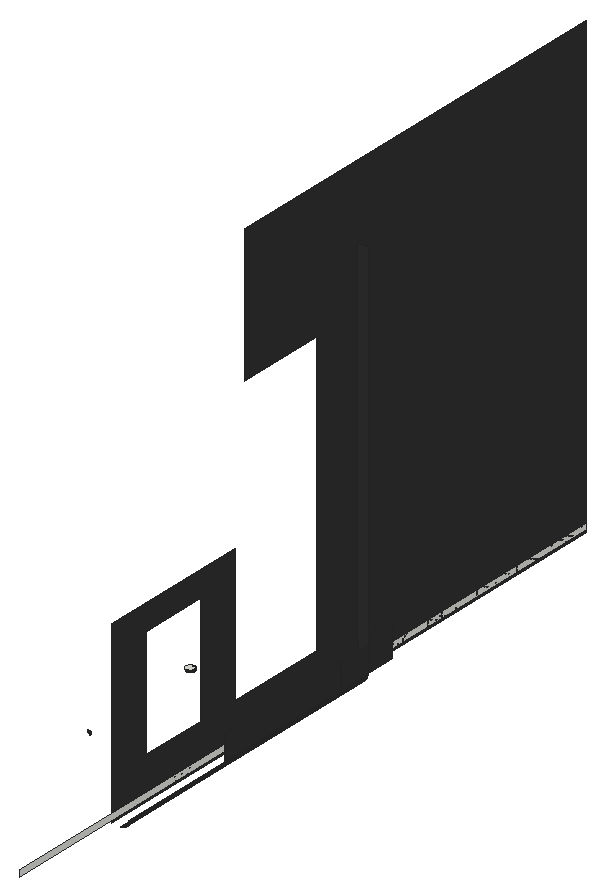
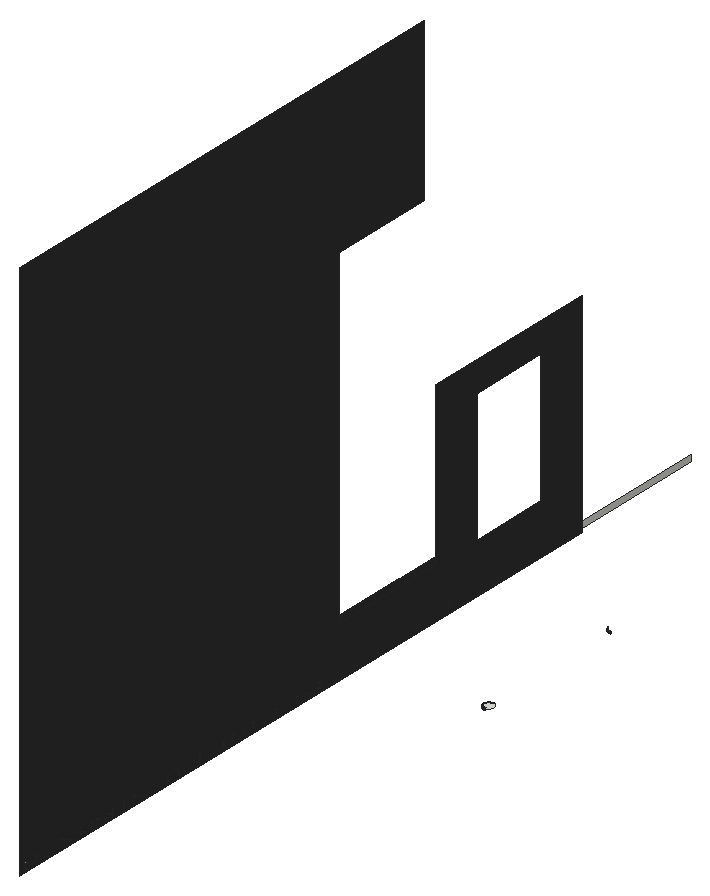
# SketchUp Ruby script. Lengths in inches.
U = 1.inch
M = Sketchup.active_model
def pt(a) = Geom::Point3d.new(a.map { |v| v * U })
def face(e, loops, mat)
  f = e.add_face(loops[0].map { |a| pt(a) })
  loops[1..].each { |l| e.add_face(l.map { |a| pt(a) }).erase! }
  f.material = f.back_material = mat if mat
  f
end
# faces: each face lists its corners as indices into pts; further lists are holes
def faces(e, pts, list, mat = nil) = list.each { |f| face(e, (f[0].is_a?(Array) ? f : [f]).map { |l| l.map { |i| pts[i] } }, mat) }
# xy, xz, yz: faces in a plane at the given z, y or x. An outline is a flat list of corners, or four numbers for a rectangle; further outlines are holes
def ring(l) = l.size == 4 ? [[l[0], l[1]], [l[2], l[1]], [l[2], l[3]], [l[0], l[3]]] : l.each_slice(2).to_a
def flat(e, list, mat, &to3) = list.each { |f| face(e, (f[0].is_a?(Array) ? f : [f]).map { |l| ring(l).map { |u, v| to3.(u, v) } }, mat) }
def xy(e, z, list, mat = nil) = flat(e, list, mat) { |x, y| [x, y, z] }
def xz(e, y, list, mat = nil) = flat(e, list, mat) { |x, z| [x, y, z] }
def yz(e, x, list, mat = nil) = flat(e, list, mat) { |y, z| [x, y, z] }
def lines(e, pts, list) = list.each { |a, b| e.add_line(pt(pts[a]), pt(pts[b])) }
# prism: a flat outline (further loops are holes) pulled along v
def prism(e, loops, v, mat = nil)
  f = face(e, loops, mat); d = Geom::Vector3d.new(v.map { |x| x * U })
  f.pushpull(f.normal.samedirection?(d) ? d.length : -d.length)
end
def box(e, o, s, mat = nil) = prism(e, [[o, [o[0] + s[0], o[1], o[2]], [o[0] + s[0], o[1] + s[1], o[2]], [o[0], o[1] + s[1], o[2]]]], [0, 0, s[2]], mat)
def at(x, y, z, deg = 0) = Geom::Transformation.translation(pt([x, y, z])) * Geom::Transformation.rotation(ORIGIN, Z_AXIS, deg.degrees)
def axes(o, x, y, z) = Geom::Transformation.new([*x, 0, *y, 0, *z, 0, *pt(o).to_a, 1])
def part(name) = M.definitions.add(name)
# library, detail: a bought-in or finely detailed component or shape, given as its bounding box
def library(name, o, s) = part(name).tap { |d| box(d.entities, o, s) }
def detail(e, o, s) = box(e.add_group.entities, o, s)
def put(e, d, t, mat = nil) = e.add_instance(d, t).tap { |i| i.material = mat if mat }
def group(e, t, mat = nil) = e.add_group.tap { |g| g.transformation = t; g.material = mat if mat }.entities
root = M.entities
M.materials.add("[Granite Dark Gray]").color = [51, 50, 50]
xy(root,126,[[438,183,438.11,393],[438.11,183,438.22,393]],"[Granite Dark Gray]")
xy(root,129,[[359.84,339,359.76,339.01,359.6875,339.02,359.61,339.03,359.45,339.05,359.375,339.07,359.3,339.08,359.22,339.1,359.15,339.125,359.07,339.15,359,339.17,358.92,339.2,358.71,339.29,358.64,339.33,358.57,339.36,358.43,339.44,358.37,339.48,358.3,339.53,358.24,339.57,358.17,339.62,357.93,339.82,357.88,339.88,357.82,339.93,357.62,340.17,357.57,340.24,357.53,340.3,357.48,340.37,357.44,340.43,357.36,340.57,357.33,340.64,357.29,340.71,357.2,340.92,357.17,341,357.15,341.07,357.125,341.15,357.1,341.22,357.08,341.3,357.07,341.375,357.05,341.45,357.03,341.61,357.02,341.6875,357.01,341.76,357,341.84,357,342.16,357.01,342.24,357.02,342.3125,357.03,342.39,357.05,342.55,357.07,342.625,357.08,342.7,357.1,342.78,357.125,342.85,357.15,342.93,357.17,343,357.2,343.08,357.29,343.29,357.33,343.36,357.36,343.43,357.44,343.57,357.48,343.63,357.53,343.7,357.57,343.76,357.62,343.83,357.82,344.07,357.88,344.12,357.93,344.18,358.17,344.38,358.24,344.43,358.3,344.47,358.37,344.52,358.43,344.56,358.57,344.64,358.64,344.67,358.71,344.71,358.92,344.8,359,344.83,359.07,344.85,359.15,344.875,359.22,344.9,359.3,344.92,359.375,344.93,359.45,344.95,359.61,344.97,359.6875,344.98,359.76,344.99,359.84,345,360.16,345,360.24,344.99,360.3125,344.98,360.39,344.97,360.55,344.95,360.625,344.93,360.7,344.92,360.78,344.9,360.85,344.875,360.93,344.85,361,344.83,361.08,344.8,361.29,344.71,361.36,344.67,361.43,344.64,361.57,344.56,361.63,344.52,361.7,344.47,361.76,344.43,361.83,344.38,362.07,344.18,362.12,344.12,362.18,344.07,362.38,343.83,362.43,343.76,362.47,343.7,362.52,343.63,362.56,343.57,362.64,343.43,362.67,343.36,362.71,343.29,362.8,343.08,362.83,343,362.85,342.93,362.875,342.85,362.9,342.78,362.92,342.7,362.93,342.625,362.95,342.55,362.97,342.39,362.98,342.3125,362.99,342.24,363,342.16,363,341.84,362.99,341.76,362.98,341.6875,362.97,341.61,362.95,341.45,362.93,341.375,362.92,341.3,362.9,341.22,362.875,341.15,362.85,341.07,362.83,341,362.8,340.92,362.71,340.71,362.67,340.64,362.64,340.57,362.56,340.43,362.52,340.37,362.47,340.3,362.43,340.24,362.38,340.17,362.18,339.93,362.12,339.88,362.07,339.82,361.83,339.62,361.76,339.57,361.7,339.53,361.63,339.48,361.57,339.44,361.43,339.36,361.36,339.33,361.29,339.29,361.08,339.2,361,339.17,360.93,339.15,360.85,339.125,360.78,339.1,360.7,339.08,360.625,339.07,360.55,339.05,360.39,339.03,360.3125,339.02,360.24,339.01,360.16,339]])
xy(root,132,[[443.875,267,444,268],[443.875,303,444,304],[443.875,369,444,370]],"[Granite Dark Gray]")
xz(root,252,[[359.84,128,359.92,129],[359.92,128,360,129],[360,128,360.08,129],[360.08,128,360.16,129]])
xz(root,267,[[443.875,132,444,150]],"[Granite Dark Gray]")
xz(root,268,[[443.875,132,444,150]],"[Granite Dark Gray]")
xz(root,303,[[443.875,132,444,150]],"[Granite Dark Gray]")
xz(root,304,[[443.875,132,444,150]],"[Granite Dark Gray]")
xz(root,339,[[359.84,128,359.92,129],[359.92,128,360,129],[360,128,360.08,129],[360.08,128,360.16,129]])
xz(root,345,[[359.84,128,359.92,129],[359.92,128,360,129],[360,128,360.08,129],[360.08,128,360.16,129]])
xz(root,369,[[443.875,132,444,150]],"[Granite Dark Gray]")
xz(root,370,[[443.875,132,444,150]],"[Granite Dark Gray]")
xz(root,393,[[437,126,437,150,436.875,150,436.875,151,437,151,437,210,436.875,210,436.875,211,437,211,437,234,436.875,234,436.875,235,437,235,437,294,436.875,294,436.875,295,437,295,437,378,436.875,378,436.875,379,437,379,437,402,444,402,444,363,443.875,363,443.875,362,444,362,444,333,443.875,333,443.875,332,444,332,444,279,443.875,279,443.875,278,444,278,444,249,443.875,249,443.875,248,444,248,444,200,443.875,200,443.875,199,444,199,444,151,443.875,151,443.875,150,444,150,444,131.78,443.95,131.23,443.93,131.12,443.92,131.01,443.9,130.9,443.85,130.68,443.83,130.57,443.8,130.46,443.77,130.36,443.74,130.25,443.71,130.15,443.67,130.04,443.63,129.9375,443.59,129.83,443.47,129.53,443.27,129.13,443.21,129.03,443.16,128.9375,443.1,128.84,442.98,128.66,442.92,128.5625,442.85,128.47,442.79,128.38,442.72,128.3,442.65,128.21,442.51,128.04,442.43,127.96,442.36,127.875,442.28,127.8,442.2,127.72,442.125,127.64,442.04,127.57,441.96,127.49,441.79,127.35,441.7,127.28,441.62,127.21,441.53,127.15,441.4375,127.08,441.34,127.02,441.16,126.9,441.0625,126.84,440.97,126.79,440.87,126.73,440.47,126.53,440.17,126.41,440.0625,126.37,439.96,126.33,439.85,126.29,439.75,126.26,439.64,126.23,439.54,126.2,439.43,126.17,439.32,126.15,439.1,126.1,438.99,126.08,438.88,126.07,438.77,126.05,438.22,126]],"[Granite Dark Gray]")
yz(root,363,[[341.84,128,341.92,129],[341.92,128,342,129],[342,128,342.08,129],[342.08,128,342.16,129]])
yz(root,432,[[102,128,600,132]])
yz(root,432,[[[183,126,183,252,291,252,291,156,363,156,363,354,300,354,300,450,600,450,600,126],[213,156,261,234]]],"[Granite Dark Gray]")
yz(root,437,[[393,126,423,150]],"[Granite Dark Gray]")
yz(root,444,[[183,131.78,393,131.89],[183,131.89,393,132],[268,132,303,150],[304,132,369,150],[370,132,393,150]],"[Granite Dark Gray]")
p = [[438.22,393,126],[438.33,393,126.01],[438.33,183,126.01],[438.22,183,126],[438.44,393,126.02],[438.44,183,126.02],
  [438.55,393,126.03],[438.55,183,126.03],[438.66,393,126.04],[438.66,183,126.04],[438.77,393,126.05],[438.77,183,126.05],
  [438.88,393,126.07],[438.88,183,126.07],[438.99,393,126.08],[438.99,183,126.08],[439.1,393,126.1],[439.1,183,126.1],
  [439.21,393,126.125],[439.21,183,126.125],[439.32,393,126.15],[439.32,183,126.15],[439.43,393,126.17],[439.43,183,126.17],
  [439.54,393,126.2],[439.54,183,126.2],[439.64,393,126.23],[439.64,183,126.23],[439.75,393,126.26],[439.75,183,126.26],
  [439.85,393,126.29],[439.85,183,126.29],[439.96,393,126.33],[439.96,183,126.33],[440.0625,393,126.37],[440.0625,183,126.37],
  [440.17,393,126.41],[440.17,183,126.41],[440.27,393,126.45],[440.27,183,126.45],[440.37,393,126.49],[440.37,183,126.49],
  [440.47,393,126.53],[440.47,183,126.53],[440.57,393,126.58],[440.57,183,126.58],[440.67,393,126.63],[440.67,183,126.63],
  [440.77,393,126.68],[440.77,183,126.68],[440.87,393,126.73],[440.87,183,126.73],[440.97,393,126.79],[440.97,183,126.79],
  [441.0625,393,126.84],[441.0625,183,126.84],[441.16,393,126.9],[441.16,183,126.9],[441.25,393,126.96],[441.25,183,126.96],
  [441.34,393,127.02],[441.34,183,127.02],[441.4375,393,127.08],[441.4375,183,127.08],[441.53,393,127.15],[441.53,183,127.15],
  [441.62,393,127.21],[441.62,183,127.21],[441.7,393,127.28],[441.7,183,127.28],[441.79,393,127.35],[441.79,183,127.35],
  [441.875,393,127.42],[441.875,183,127.42],[441.96,393,127.49],[441.96,183,127.49],[442.04,393,127.57],[442.04,183,127.57],
  [442.125,393,127.64],[442.125,183,127.64],[442.2,393,127.72],[442.2,183,127.72],[442.28,393,127.8],[442.28,183,127.8],
  [442.36,393,127.875],[442.36,183,127.875],[442.43,393,127.96],[442.43,183,127.96],[442.51,393,128.04],[442.51,183,128.04],
  [442.58,393,128.125],[442.58,183,128.125],[362.92,249.7,128],[362.93,249.625,128],[362.93,249.625,129],[362.92,249.7,129],
  [362.9,249.78,128],[362.9,249.78,129],[362.875,249.85,128],[362.875,249.85,129],[362.83,250,128],[362.85,249.93,128],
  [362.85,249.93,129],[362.83,250,129],[362.8,250.08,128],[362.8,250.08,129],[362.74,250.22,128],[362.77,250.15,128],
  [362.77,250.15,129],[362.74,250.22,129],[362.71,250.29,128],[362.71,250.29,129],[362.67,250.36,128],[362.67,250.36,129],
  [362.64,250.43,128],[362.64,250.43,129],[362.6,250.5,128],[362.6,250.5,129],[362.56,250.57,128],[362.56,250.57,129],
  [362.52,250.63,128],[362.52,250.63,129],[362.47,250.7,128],[362.47,250.7,129],[362.43,250.76,128],[362.43,250.76,129],
  [362.33,250.89,128],[362.38,250.83,128],[362.38,250.83,129],[362.33,250.89,129],[362.23,251.01,128],[362.28,250.95,128],
  [362.28,250.95,129],[362.23,251.01,129],[362.18,251.07,128],[362.18,251.07,129],[362.12,251.12,128],[362.12,251.12,129],
  [362.07,251.18,128],[362.07,251.18,129],[361.95,251.28,128],[362.01,251.23,128],[362.01,251.23,129],[361.95,251.28,129],
  [361.83,251.38,128],[361.89,251.33,128],[361.89,251.33,129],[361.83,251.38,129],[361.7,251.47,128],[361.76,251.43,128],
  [361.76,251.43,129],[361.7,251.47,129],[361.63,251.52,128],[361.63,251.52,129],[361.57,251.56,128],[361.57,251.56,129],
  [361.43,251.64,128],[361.5,251.6,128],[361.5,251.6,129],[361.43,251.64,129],[361.36,251.67,128],[361.36,251.67,129],
  [361.15,251.77,128],[361.22,251.74,128],[361.22,251.74,129],[361.15,251.77,129],[361.29,251.71,128],[361.29,251.71,129],
  [360.93,251.85,128],[361,251.83,128],[361,251.83,129],[360.93,251.85,129],[361.08,251.8,128],[361.08,251.8,129],
  [359.375,251.93,128],[359.45,251.95,128],[359.45,251.95,129],[359.375,251.93,129],[359.53,251.96,128],[359.53,251.96,129],
  [360.55,251.95,128],[360.625,251.93,128],[360.625,251.93,129],[360.55,251.95,129],[360.47,251.96,128],[360.47,251.96,129],
  [360.7,251.92,128],[360.7,251.92,129],[360.78,251.9,128],[360.78,251.9,129],[360.85,251.875,128],[360.85,251.875,129],
  [359.61,251.97,128],[359.61,251.97,129],[359.6875,251.98,128],[359.6875,251.98,129],[359.76,251.99,128],[359.76,251.99,129],
  [359.84,252,128],[359.84,252,129],[360.24,251.99,128],[360.3125,251.98,128],[360.3125,251.98,129],[360.24,251.99,129],
  [360.16,252,128],[360.16,252,129],[360.39,251.97,128],[360.39,251.97,129],[359.61,339.03,128],[359.53,339.04,128],
  [359.53,339.04,129],[359.61,339.03,129],[359.45,339.05,128],[359.45,339.05,129],[359.6875,339.02,128],[359.6875,339.02,129],
  [359.76,339.01,128],[359.76,339.01,129],[359.84,339,128],[359.84,339,129],[360.24,339.01,128],[360.16,339,128],
  [360.16,339,129],[360.24,339.01,129],[360.3125,339.02,128],[360.3125,339.02,129],[360.39,339.03,128],[360.39,339.03,129],
  [360.47,339.04,128],[360.47,339.04,129],[360.55,339.05,128],[360.55,339.05,129],[359.375,339.07,128],[359.3,339.08,128],
  [359.3,339.08,129],[359.375,339.07,129],[360.625,339.07,128],[360.625,339.07,129],[360.7,339.08,128],[360.7,339.08,129],
  [360.78,339.1,128],[360.78,339.1,129],[360.85,339.125,128],[360.85,339.125,129],[360.93,339.15,128],[360.93,339.15,129],
  [361,339.17,128],[361,339.17,129],[361.08,339.2,128],[361.08,339.2,129],[361.15,339.23,128],[361.15,339.23,129],
  [361.22,339.26,128],[361.22,339.26,129],[361.29,339.29,128],[361.29,339.29,129],[361.36,339.33,128],[361.36,339.33,129],
  [361.43,339.36,128],[361.43,339.36,129],[361.5,339.4,128],[361.5,339.4,129],[361.57,339.44,128],[361.57,339.44,129],
  [361.63,339.48,128],[361.63,339.48,129],[361.7,339.53,128],[361.7,339.53,129],[361.76,339.57,128],[361.76,339.57,129],
  [361.83,339.62,128],[361.83,339.62,129],[361.89,339.67,128],[361.89,339.67,129],[361.95,339.72,128],[361.95,339.72,129],
  [362.01,339.77,128],[362.01,339.77,129],[362.07,339.82,128],[362.07,339.82,129],[362.12,339.88,128],[362.12,339.88,129],
  [362.18,339.93,128],[362.18,339.93,129],[362.23,339.99,128],[362.23,339.99,129],[362.28,340.05,128],[362.28,340.05,129],
  [362.33,340.11,128],[362.33,340.11,129],[362.38,340.17,128],[362.38,340.17,129],[362.43,340.24,128],[362.43,340.24,129],
  [362.47,340.3,128],[362.47,340.3,129],[362.52,340.37,128],[362.52,340.37,129],[362.56,340.43,128],[362.56,340.43,129],
  [362.6,340.5,128],[362.6,340.5,129],[362.64,340.57,128],[362.64,340.57,129],[362.67,340.64,128],[362.67,340.64,129],
  [362.71,340.71,128],[362.71,340.71,129],[362.74,340.78,128],[362.74,340.78,129],[362.77,340.85,128],[362.77,340.85,129],
  [362.8,340.92,128],[362.8,340.92,129],[362.83,341,128],[362.83,341,129],[362.85,341.07,128],[362.85,341.07,129],
  [362.875,341.15,128],[362.875,341.15,129],[362.9,341.22,128],[362.9,341.22,129],[362.92,341.3,128],[362.92,341.3,129],
  [362.93,341.375,128],[362.93,341.375,129],[362.95,341.45,128],[362.95,341.45,129],[362.96,341.53,128],[362.96,341.53,129],
  [362.97,341.61,128],[362.97,341.61,129],[362.98,341.6875,128],[362.98,341.6875,129],[362.99,341.76,128],[362.99,341.76,129],
  [363,341.84,128],[363,341.84,129],[362.99,342.24,128],[363,342.16,128],[363,342.16,129],[362.99,342.24,129],
  [362.98,342.3125,128],[362.98,342.3125,129],[362.97,342.39,128],[362.97,342.39,129],[362.96,342.47,128],[362.96,342.47,129],
  [362.95,342.55,128],[362.95,342.55,129],[362.93,342.625,128],[362.93,342.625,129],[362.92,342.7,128],[362.92,342.7,129],
  [362.9,342.78,128],[362.9,342.78,129],[362.875,342.85,128],[362.875,342.85,129],[362.83,343,128],[362.85,342.93,128],
  [362.85,342.93,129],[362.83,343,129],[362.8,343.08,128],[362.8,343.08,129],[362.74,343.22,128],[362.77,343.15,128],
  [362.77,343.15,129],[362.74,343.22,129],[362.71,343.29,128],[362.71,343.29,129],[362.67,343.36,128],[362.67,343.36,129],
  [362.64,343.43,128],[362.64,343.43,129],[362.6,343.5,128],[362.6,343.5,129],[362.56,343.57,128],[362.56,343.57,129],
  [362.52,343.63,128],[362.52,343.63,129],[362.47,343.7,128],[362.47,343.7,129],[362.43,343.76,128],[362.43,343.76,129],
  [362.33,343.89,128],[362.38,343.83,128],[362.38,343.83,129],[362.33,343.89,129],[362.23,344.01,128],[362.28,343.95,128],
  [362.28,343.95,129],[362.23,344.01,129],[362.18,344.07,128],[362.18,344.07,129],[362.12,344.12,128],[362.12,344.12,129],
  [362.07,344.18,128],[362.07,344.18,129],[361.95,344.28,128],[362.01,344.23,128],[362.01,344.23,129],[361.95,344.28,129],
  [361.83,344.38,128],[361.89,344.33,128],[361.89,344.33,129],[361.83,344.38,129],[361.7,344.47,128],[361.76,344.43,128],
  [361.76,344.43,129],[361.7,344.47,129],[361.63,344.52,128],[361.63,344.52,129],[361.57,344.56,128],[361.57,344.56,129],
  [361.43,344.64,128],[361.5,344.6,128],[361.5,344.6,129],[361.43,344.64,129],[361.36,344.67,128],[361.36,344.67,129],
  [361.15,344.77,128],[361.22,344.74,128],[361.22,344.74,129],[361.15,344.77,129],[361.29,344.71,128],[361.29,344.71,129],
  [360.93,344.85,128],[361,344.83,128],[361,344.83,129],[360.93,344.85,129],[361.08,344.8,128],[361.08,344.8,129],
  [359.375,344.93,128],[359.45,344.95,128],[359.45,344.95,129],[359.375,344.93,129],[359.53,344.96,128],[359.53,344.96,129],
  [360.55,344.95,128],[360.625,344.93,128],[360.625,344.93,129],[360.55,344.95,129],[360.47,344.96,128],[360.47,344.96,129],
  [360.7,344.92,128],[360.7,344.92,129],[360.78,344.9,128],[360.78,344.9,129],[360.85,344.875,128],[360.85,344.875,129],
  [359.61,344.97,128],[359.61,344.97,129],[359.6875,344.98,128],[359.6875,344.98,129],[359.76,344.99,128],[359.76,344.99,129],
  [359.84,345,128],[359.84,345,129],[360.24,344.99,128],[360.3125,344.98,128],[360.3125,344.98,129],[360.24,344.99,129],
  [360.16,345,128],[360.16,345,129],[360.39,344.97,128],[360.39,344.97,129],[442.65,393,128.21],[442.65,183,128.21],
  [442.72,393,128.3],[442.72,183,128.3],[442.79,393,128.38],[442.79,183,128.38],[442.85,393,128.47],[442.85,183,128.47],
  [442.92,393,128.5625],[442.92,183,128.5625],[442.98,393,128.66],[442.98,183,128.66],[443.04,393,128.75],[443.04,183,128.75],
  [443.1,393,128.84],[443.1,183,128.84],[443.16,393,128.9375],[443.16,183,128.9375],[443.21,393,129.03],[443.21,183,129.03],
  [443.27,393,129.13],[443.27,183,129.13],[443.32,393,129.23],[443.32,183,129.23],[443.37,393,129.33],[443.37,183,129.33],
  [443.42,393,129.43],[443.42,183,129.43],[443.47,393,129.53],[443.47,183,129.53],[443.51,393,129.63],[443.51,183,129.63],
  [443.55,393,129.73],[443.55,183,129.73],[443.59,393,129.83],[443.59,183,129.83],[443.63,393,129.9375],[443.63,183,129.9375],
  [443.67,393,130.04],[443.67,183,130.04],[443.71,393,130.15],[443.71,183,130.15],[443.74,393,130.25],[443.74,183,130.25],
  [443.77,393,130.36],[443.77,183,130.36],[443.8,393,130.46],[443.8,183,130.46],[443.83,393,130.57],[443.83,183,130.57],
  [443.85,393,130.68],[443.85,183,130.68],[443.875,393,130.79],[443.875,183,130.79],[443.9,393,130.9],[443.9,183,130.9],
  [443.92,393,131.01],[443.92,183,131.01],[443.93,393,131.12],[443.93,183,131.12],[443.95,393,131.23],[443.95,183,131.23],
  [443.96,393,131.34],[443.96,183,131.34],[443.97,393,131.45],[443.97,183,131.45],[443.98,393,131.56],[443.98,183,131.56],
  [443.99,393,131.67],[443.99,183,131.67],[444,393,131.78],[444,183,131.78]]
faces(root,p,[[0,1,2,3],[1,4,5,2],[4,6,7,5],[6,8,9,7],[8,10,11,9],[10,12,13,11],[12,14,15,13],[14,16,17,15],
  [16,18,19,17],[18,20,21,19],[20,22,23,21],[22,24,25,23],[24,26,27,25],[26,28,29,27],[28,30,31,29],[30,32,33,31],
  [32,34,35,33],[34,36,37,35],[36,38,39,37],[38,40,41,39],[40,42,43,41],[42,44,45,43],[44,46,47,45],[46,48,49,47],
  [48,50,51,49],[50,52,53,51],[52,54,55,53],[54,56,57,55],[56,58,59,57],[58,60,61,59],[60,62,63,61],[62,64,65,63],
  [64,66,67,65],[66,68,69,67],[68,70,71,69],[70,72,73,71],[72,74,75,73],[74,76,77,75],[76,78,79,77],[78,80,81,79],
  [80,82,83,81],[82,84,85,83],[84,86,87,85],[86,88,89,87],[88,90,91,89],[90,466,467,91],[466,468,469,467],[468,470,471,469],
  [470,472,473,471],[472,474,475,473],[474,476,477,475],[476,478,479,477],[478,480,481,479],[480,482,483,481],[482,484,485,483],[484,486,487,485],
  [486,488,489,487],[488,490,491,489],[490,492,493,491],[492,494,495,493],[494,496,497,495],[496,498,499,497],[498,500,501,499],[500,502,503,501],
  [502,504,505,503],[504,506,507,505],[506,508,509,507],[508,510,511,509],[510,512,513,511],[512,514,515,513],[514,516,517,515],[516,518,519,517],
  [518,520,521,519],[520,522,523,521],[522,524,525,523],[524,526,527,525],[526,528,529,527],[528,530,531,529],[530,532,533,531],[532,534,535,533],
  [534,536,537,535]],"[Granite Dark Gray]")
faces(root,p,[[92,93,94,95],[96,92,95,97],[98,96,97,99],[100,101,102,103],[101,98,99,102],[104,100,103,105],[106,107,108,109],[107,104,105,108],
  [110,106,109,111],[112,110,111,113],[114,112,113,115],[116,114,115,117],[118,116,117,119],[120,118,119,121],[122,120,121,123],[124,122,123,125],
  [126,127,128,129],[127,124,125,128],[130,131,132,133],[131,126,129,132],[134,130,133,135],[136,134,135,137],[138,136,137,139],[140,141,142,143],
  [141,138,139,142],[144,145,146,147],[145,140,143,146],[148,149,150,151],[149,144,147,150],[152,148,151,153],[154,152,153,155],[156,157,158,159],
  [160,156,159,161],[157,154,155,158],[162,163,164,165],[163,166,167,164],[166,160,161,167],[168,169,170,171],[169,172,173,170],[172,162,165,173],
  [174,175,176,177],[175,178,179,176],[180,181,182,183],[184,180,183,185],[181,186,187,182],[186,188,189,187],[188,190,191,189],[190,168,171,191],
  [178,192,193,179],[192,194,195,193],[194,196,197,195],[196,198,199,197],[200,201,202,203],[204,200,203,205],[201,206,207,202],[206,184,185,207],
  [208,209,210,211],[209,212,213,210],[214,208,211,215],[216,214,215,217],[218,216,217,219],[220,221,222,223],[224,220,223,225],[226,224,225,227],
  [228,226,227,229],[230,228,229,231],[232,233,234,235],[212,232,235,213],[236,230,231,237],[238,236,237,239],[240,238,239,241],[242,240,241,243],
  [244,242,243,245],[246,244,245,247],[248,246,247,249],[250,248,249,251],[252,250,251,253],[254,252,253,255],[256,254,255,257],[258,256,257,259],
  [260,258,259,261],[262,260,261,263],[264,262,263,265],[266,264,265,267],[268,266,267,269],[270,268,269,271],[272,270,271,273],[274,272,273,275],
  [276,274,275,277],[278,276,277,279],[280,278,279,281],[282,280,281,283],[284,282,283,285],[286,284,285,287],[288,286,287,289],[290,288,289,291],
  [292,290,291,293],[294,292,293,295],[296,294,295,297],[298,296,297,299],[300,298,299,301],[302,300,301,303],[304,302,303,305],[306,304,305,307],
  [308,306,307,309],[310,308,309,311],[312,310,311,313],[314,312,313,315],[316,314,315,317],[318,316,317,319],[320,318,319,321],[322,320,321,323],
  [324,322,323,325],[326,324,325,327],[328,326,327,329],[330,328,329,331],[332,330,331,333],[334,332,333,335],[336,334,335,337],[338,339,340,341],
  [342,338,341,343],[344,342,343,345],[346,344,345,347],[348,346,347,349],[350,348,349,351],[352,350,351,353],[354,352,353,355],[356,354,355,357],
  [358,359,360,361],[359,356,357,360],[362,358,361,363],[364,365,366,367],[365,362,363,366],[368,364,367,369],[370,368,369,371],[372,370,371,373],
  [374,372,373,375],[376,374,375,377],[378,376,377,379],[380,378,379,381],[382,380,381,383],[384,385,386,387],[385,382,383,386],[388,389,390,391],
  [389,384,387,390],[392,388,391,393],[394,392,393,395],[396,394,395,397],[398,399,400,401],[399,396,397,400],[402,403,404,405],[403,398,401,404],
  [406,407,408,409],[407,402,405,408],[410,406,409,411],[412,410,411,413],[414,415,416,417],[418,414,417,419],[415,412,413,416],[420,421,422,423],
  [421,424,425,422],[424,418,419,425],[426,427,428,429],[427,430,431,428],[430,420,423,431],[432,433,434,435],[433,436,437,434],[438,439,440,441],
  [442,438,441,443],[439,444,445,440],[444,446,447,445],[446,448,449,447],[448,426,429,449],[436,450,451,437],[450,452,453,451],[452,454,455,453],
  [454,456,457,455],[458,459,460,461],[462,458,461,463],[459,464,465,460],[464,442,443,465]])
